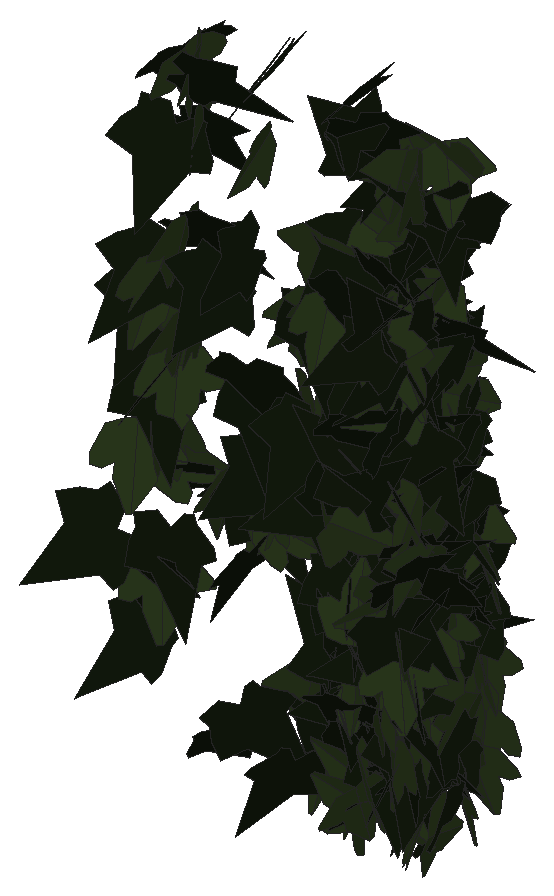
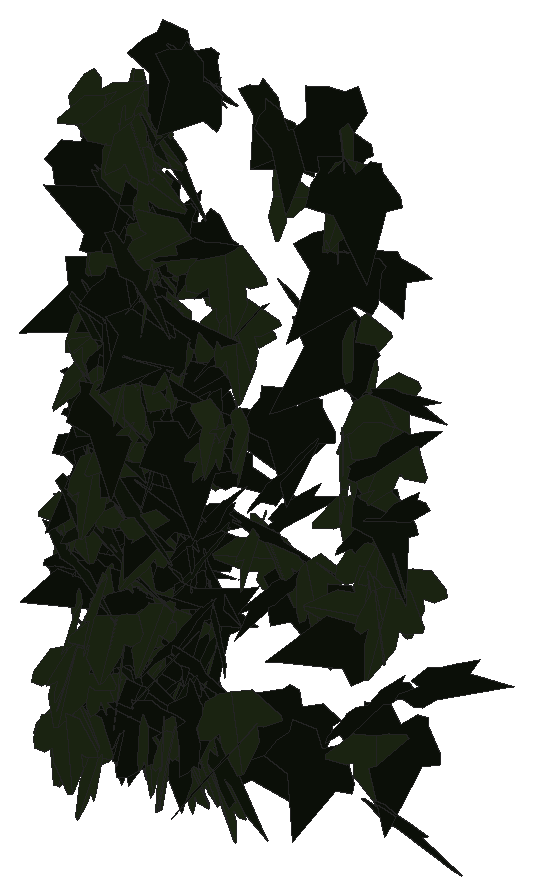
# SketchUp Ruby script. Lengths in inches.
U = 1.inch
M = Sketchup.active_model
def pt(a) = Geom::Point3d.new(a.map { |v| v * U })
def face(e, loops, mat)
  f = e.add_face(loops[0].map { |a| pt(a) })
  loops[1..].each { |l| e.add_face(l.map { |a| pt(a) }).erase! }
  f.material = f.back_material = mat if mat
  f
end
# faces: each face lists its corners as indices into pts; further lists are holes
def faces(e, pts, list, mat = nil) = list.each { |f| face(e, (f[0].is_a?(Array) ? f : [f]).map { |l| l.map { |i| pts[i] } }, mat) }
# xy, xz, yz: faces in a plane at the given z, y or x. An outline is a flat list of corners, or four numbers for a rectangle; further outlines are holes
def ring(l) = l.size == 4 ? [[l[0], l[1]], [l[2], l[1]], [l[2], l[3]], [l[0], l[3]]] : l.each_slice(2).to_a
def flat(e, list, mat, &to3) = list.each { |f| face(e, (f[0].is_a?(Array) ? f : [f]).map { |l| ring(l).map { |u, v| to3.(u, v) } }, mat) }
def xy(e, z, list, mat = nil) = flat(e, list, mat) { |x, y| [x, y, z] }
def xz(e, y, list, mat = nil) = flat(e, list, mat) { |x, z| [x, y, z] }
def yz(e, x, list, mat = nil) = flat(e, list, mat) { |y, z| [x, y, z] }
def lines(e, pts, list) = list.each { |a, b| e.add_line(pt(pts[a]), pt(pts[b])) }
# prism: a flat outline (further loops are holes) pulled along v
def prism(e, loops, v, mat = nil)
  f = face(e, loops, mat); d = Geom::Vector3d.new(v.map { |x| x * U })
  f.pushpull(f.normal.samedirection?(d) ? d.length : -d.length)
end
def box(e, o, s, mat = nil) = prism(e, [[o, [o[0] + s[0], o[1], o[2]], [o[0] + s[0], o[1] + s[1], o[2]], [o[0], o[1] + s[1], o[2]]]], [0, 0, s[2]], mat)
def at(x, y, z, deg = 0) = Geom::Transformation.translation(pt([x, y, z])) * Geom::Transformation.rotation(ORIGIN, Z_AXIS, deg.degrees)
def axes(o, x, y, z) = Geom::Transformation.new([*x, 0, *y, 0, *z, 0, *pt(o).to_a, 1])
def part(name) = M.definitions.add(name)
# library, detail: a bought-in or finely detailed component or shape, given as its bounding box
def library(name, o, s) = part(name).tap { |d| box(d.entities, o, s) }
def detail(e, o, s) = box(e.add_group.entities, o, s)
def put(e, d, t, mat = nil) = e.add_instance(d, t).tap { |i| i.material = mat if mat }
def group(e, t, mat = nil) = e.add_group.tap { |g| g.transformation = t; g.material = mat if mat }.entities
root = M.entities
M.materials.add("efeu1").color = [18, 25, 13]
M.materials.add("efeu2").color = [43, 57, 29]
c1 = part("ivyleaf_9")
p = [[1.54,2.16,1.25],[1.36,2.04,1.19],[-0.21,0.99,0.68],[-0.71,1.11,0.82],[-0.85,0.86,0.67],[-0.8,0.17,0.21],
  [-0.9,-0.01,0.1],[-0.67,-0.16,-0.02],[-0.08,-0.08,-0.05],[-0.03,-0.6,-0.4],[0.65,-0.88,-0.66],[0.83,-0.6,-0.49],
  [1.29,-0.42,-0.43],[1.8125,-0.07,-0.26],[1.21,0.44,0.15]]
faces(c1.entities,p,[[0,1,2,3,4,5,6,7,8,9,10,11,12,13,14]],"efeu1")
c2 = part("ivyleaf_10")
p = [[0,0.5,-0.03],[-0.0625,2.02,-0.43],[-0.19,2.01,-0.46],[-0.54,1.05,-0.29],[-0.52,0.625,-0.18],[-0.83,0.76,-0.28],
  [-1.16,0.64,-0.33],[-1.15,0.33,-0.24],[-0.77,-0.39,0.02],[-0.3,-0.51,0.16],[0.04,-0.48,0.23],[-0.02,2.01,-0.4375],
  [-0.06,2.01,-0.43],[0.04,-0.49,0.23],[0.67,-0.49,0.14],[1.38,0.36,-0.2],[1.375,0.51,-0.24],[0.81,0.65,-0.19],
  [0.62,0.59,-0.15],[0.6,1.09,-0.28],[0.5,1.23,-0.31]]
faces(c2.entities,p,[[0,1,2,3,4,5,6,7,8,9,10],[11,12,0,13,14,15,16,17,18,19,20]],"efeu2")
put(root,c1,axes([2.26,224.04,225.46],[-0.33992,-0.24824,0.26986],[-0.17412,-0.21457,-0.4167],[0.3227,-0.37727,0.05943]))
put(root,c1,axes([2.4,224.73,223.76],[-0.49927,0.02483,-0.01047],[0.00793,-0.05019,-0.49741],[-0.02575,-0.49685,0.04972]))
put(root,c1,axes([2.41,224.39,224.89],[0.35781,0.24755,-0.24635],[-0.21533,-0.1213,-0.43465],[-0.27496,0.41714,0.0198]))
put(root,c2,axes([2.41,224.64,226.9],[-0.10833,-0.43935,-0.21269],[0.08333,0.19802,-0.45149],[0.48096,-0.13327,0.03032]))
put(root,c2,axes([2.68,224.61,227.07],[0.27047,-0.37993,-0.18027],[-0.08089,0.16333,-0.4656],[0.41268,0.28102,0.02689]))
put(root,c2,axes([2.55,224.69,224.7],[0.37414,0.33148,0.01172],[0.00935,0.00712,-0.49986],[-0.33156,0.37426,-0.00086]))
put(root,c2,axes([2.63,224.04,226.96],[0.42358,0.26564,-0.00356],[-0.00319,-0.00162,-0.49999],[-0.26565,0.42359,0.00033]))
put(root,c1,axes([2.74,224.42,229.04],[-0.21253,-0.4395,0.10803],[-0.03639,-0.10236,-0.48806],[0.45112,-0.21531,0.01152]))
put(root,c1,axes([3.02,223.99,228.01],[-0.17079,0.46892,0.03075],[-0.00354,0.03144,-0.499],[-0.46991,-0.17067,-0.00742]))
put(root,c2,axes([2.91,224.34,227.25],[-0.49705,0.04613,0.02857],[-0.03096,-0.02493,-0.49842],[-0.04456,-0.49724,0.02763]))
put(root,c1,axes([2.7,224.7,225.29],[0.04335,-0.49242,-0.07509],[-0.00716,0.07475,-0.49433],[0.49807,0.04393,-0.00057]))
put(root,c2,axes([2.96,224.12,227.24],[-0.17393,0.43653,0.17084],[-0.13153,0.12946,-0.46469],[-0.44994,-0.20659,0.0698]))
put(root,c1,axes([3.02,224.12,229.75],[-0.4399,-0.23646,0.02393],[0.03632,-0.11663,-0.48485],[0.23487,-0.42484,0.11979]))
put(root,c2,axes([2.88,224.1,229.02],[-0.44475,-0.18072,-0.13976],[0.1366,0.03482,-0.47972],[0.18312,-0.46489,0.0184]))
put(root,c1,axes([2.87,224.22,227.9],[-0.00625,-0.48515,-0.12079],[-0.01142,0.1209,-0.48503],[0.49983,-0.0033,-0.0126]))
put(root,c2,axes([3.09,223.94,229.59],[0.20409,0.4084,-0.20385],[-0.1269,-0.16372,-0.45507],[-0.43845,0.23749,0.03683]))
put(root,c2,axes([2.77,224.45,226.53],[0.00807,-0.03471,0.49873],[0.43105,0.25315,0.01064],[-0.25324,0.42978,0.03401]))
put(root,c1,axes([2.82,224.54,226.32],[0.44308,0.01063,0.23144],[0.22107,0.13005,-0.4292],[-0.06932,0.48267,0.11055]))
put(root,c2,axes([3.11,224.3125,228.08],[0.31685,0.38417,-0.04498],[-0.03416,-0.03013,-0.49792],[-0.38528,0.3186,0.00715]))
put(root,c1,axes([3.35,224.15,233.01],[0.01762,0.49548,-0.06469],[-0.05228,-0.06255,-0.49331],[-0.49695,0.02415,0.04961]))
put(root,c1,axes([3.21,224.11,231.76],[-0.38608,-0.29312,-0.12255],[0.09909,0.07214,-0.48474],[0.30186,-0.39859,0.00239]))
put(root,c2,axes([3.26,224.27,228.88],[0.04513,-0.49718,-0.02777],[0.00392,0.02824,-0.49919],[0.49794,0.04484,0.00644]))
put(root,c2,axes([3.38,224.36,228.92],[0.20097,-0.39637,-0.22913],[-0.02558,0.24012,-0.43782],[0.45712,0.1877,0.07624]))
put(root,c2,axes([3.42,224.02,230.4],[0.06062,-0.49609,0.01495],[0.01955,-0.01266,-0.49946],[0.49593,0.06114,0.01786]))
put(root,c1,axes([3.26,224.29,231.83],[0.46235,0.1903,0.00424],[0.00518,-0.00145,-0.49997],[-0.19027,0.46237,-0.00332]))
put(root,c2,axes([3.47,224.09,232.91],[-0.16037,-0.41396,-0.23004],[0.10967,0.20381,-0.44321],[0.46071,-0.19261,0.02543]))
put(root,c2,axes([3.73,223.97,232.07],[-0.1549,0.42725,0.20849],[-0.26925,0.10187,-0.40881],[-0.3918,-0.23892,0.19851]))
put(root,c1,axes([3.47,224.12,230.39],[0.47347,0.14341,0.0725],[0.0648,0.03605,-0.49447],[-0.14705,0.47763,0.01555]))
put(root,c2,axes([3.81,223.8,233.15],[0.22729,-0.43822,-0.07937],[0.0098,0.09401,-0.49099],[0.44525,0.22164,0.05132]))
put(root,c2,axes([3.9,224.42,226.68],[0.05666,-0.49677,-0.00238],[-0.00053,0.00234,-0.49999],[0.49678,0.05666,-0.00027]))
put(root,c1,axes([4.08,224.09,229.77],[-0.22286,-0.3816,0.23391],[0.00769,-0.26453,-0.42422],[0.44752,-0.18549,0.12377]))
put(root,c1,axes([4.42,223.59,223.47],[0.16265,0.40557,0.04719],[0.02659,0.03925,-0.44983],[-0.43994,0.15232,-0.00974]))
put(root,c1,axes([4.06,223.4,233.14],[0.44335,0.04612,0.22652],[0.22564,0.02018,-0.44574],[-0.05026,0.49746,-0.00292]))
put(root,c1,axes([4.69,223.84,230.5625],[-0.44518,0.11169,-0.086],[0.08585,-0.02281,-0.44415],[-0.1231,-0.4198,0.00125]))
put(root,c1,axes([4.31,224.49,226.55],[0.16793,-0.41956,-0.21393],[-0.00025,0.22705,-0.44548],[0.47096,0.14972,0.07605]))
put(root,c1,axes([4.96,224.46,227.18],[-0.45656,0.1186,0.16579],[-0.18044,-0.04595,-0.46404],[-0.09484,-0.48355,0.08476]))
put(root,c1,axes([4.75,223.74,226.1],[-0.14471,0.36375,-0.20527],[0.07559,-0.18455,-0.40315],[-0.44052,-0.15116,-0.00175]))
put(root,c1,axes([4.78,223.85,233.08],[-0.06579,0.3891,0.19208],[-0.01428,0.18475,-0.40934],[-0.46495,-0.06073,-0.01461]))
put(root,c1,axes([4.66,223.83,228.81],[0.32779,0.22367,-0.22565],[-0.18782,-0.12974,-0.39211],[-0.27926,0.34981,-0.00115]))
put(root,c1,axes([4.43,224.33,228.15],[0.07692,-0.49391,0.01152],[-0.0076,-0.01284,-0.49978],[0.49399,0.07671,-0.00948]))
put(root,c1,axes([4.8,224.06,227.16],[-0.21161,-0.24551,0.31297],[-0.13765,-0.27775,-0.32196],[0.39622,-0.22761,0.0553]))
put(root,c2,axes([4.85,224.0625,226.75],[0.42955,-0.14661,-0.10158],[-0.09536,0.0428,-0.44074],[0.16463,0.40731,0.00975]))
put(root,c2,axes([4.85,223.95,232.14],[-0.07874,0.19352,-0.39801],[-0.08017,-0.38802,-0.18936],[-0.45616,0.03479,0.10198]))
put(root,c1,axes([4.96,223.8125,233.24],[0.0911,0.29753,0.31816],[-0.01364,0.31344,-0.31342],[-0.46068,0.04956,0.0722]))
put(root,c1,axes([4.85,223.51,223.96],[-0.04578,-0.12272,-0.43178],[0.14281,0.39355,-0.13503],[0.44522,-0.13886,-0.00109]))
put(root,c2,axes([5.05,224.18,226.94],[-0.15635,0.40635,0.05835],[-0.02651,0.05081,-0.44858],[-0.44222,-0.14671,0.00626]))
put(root,c2,axes([5.28,224.41,224.2],[-0.31464,-0.31848,0.05623],[-0.03611,-0.04269,-0.44887],[0.347,-0.29322,0.00428]))
put(root,c2,axes([5.15,224.375,228.47],[-0.26711,0.29156,-0.21578],[0.10472,-0.18818,-0.39521],[-0.37202,-0.26231,0.04369]))
put(root,c1,axes([5.41,224.51,223.39],[-0.34283,0.23911,-0.18396],[0.14872,-0.11116,-0.41327],[-0.28472,-0.34597,0.00564]))
put(root,c2,axes([4.92,223.98,226.49],[0.09282,0.01907,0.44304],[0.42676,0.1598,-0.09035],[-0.17312,0.40414,0.01482]))
put(root,c1,axes([5.14,224.7,223.66],[0.28128,-0.3725,-0.17923],[-0.05231,0.18297,-0.46237],[0.41005,0.27887,0.06396]))
put(root,c2,axes([5.54,224.48,228.54],[0.07507,0.17716,0.40681],[-0.28386,0.33091,-0.10729],[-0.36674,-0.21986,0.16631]))
put(root,c2,axes([5.47,224.08,229.875],[-0.02902,-0.49379,-0.07302],[0.00703,0.07273,-0.49463],[0.49911,-0.02974,0.00273]))
put(root,c2,axes([5.39,224.54,223.06],[0.40203,-0.22472,0.01308],[0.01328,-0.00397,-0.4522],[0.24271,0.37244,0.00307]))
put(root,c1,axes([5.57,223.64,223.32],[-0.04818,0.25155,-0.36616],[0.02111,-0.35241,-0.26444],[-0.46685,-0.04189,0.02583]))
put(root,c2,axes([5.56,224.16,229.99],[-0.23399,-0.43296,0.08831],[-0.01094,-0.09422,-0.49092],[0.44174,-0.23167,0.03462]))
put(root,c2,axes([5.6875,224.12,230.85],[-0.47361,-0.09232,0.13103],[-0.12689,-0.03378,-0.48245],[0.09793,-0.49024,0.00857]))
put(root,c2,axes([5.52,224.46,228.32],[-0.04509,0.41578,0.1257],[-0.00059,0.12137,-0.43443],[-0.46763,-0.04024,-0.01157]))
put(root,c1,axes([5.73,223.8,228.29],[-0.40757,-0.20368,-0.07589],[0.0698,0.03389,-0.44599],[0.223,-0.38287,0.0009]))
put(root,c1,axes([5.51,224.15,229.75],[0.10925,-0.48418,0.06029],[0.01544,-0.05832,-0.49635],[0.48767,0.11031,0.00221]))
put(root,c1,axes([5.875,224.62,228.23],[0.06639,0.42206,-0.08893],[-0.01441,-0.08446,-0.44357],[-0.46486,0.0629,0.00105]))
put(root,c2,axes([5.93,225.01,223.7],[-0.289,0.25274,0.2411],[-0.17101,0.16978,-0.38258],[-0.32856,-0.31068,-0.01294]))
put(root,c1,axes([6.19,223.71,227.4],[-0.40656,-0.02731,0.22492],[-0.23282,-0.01735,-0.39253],[0.03491,-0.4338,0.00154]))
put(root,c1,axes([6.24,224.47,229.82],[-0.11263,0.17983,0.3974],[-0.37704,0.18477,-0.18952],[-0.25665,-0.35035,0.10402]))
put(root,c1,axes([5.59,224.86,224],[0.12589,-0.03447,-0.43438],[0.45055,-0.03188,0.12381],[-0.04325,-0.43246,0.0255]))
put(root,c1,axes([6.07,223.7,224.7],[0.07921,-0.04203,0.44378],[-0.0227,0.43203,0.04801],[-0.46252,-0.0284,0.07365]))
put(root,c2,axes([6.21,223.94,223.01],[0.16723,-0.11354,-0.40594],[-0.26434,0.30745,-0.19398],[0.35053,0.28602,0.04738]))
put(root,c1,axes([5.87,224.42,226.79],[-0.0248,-0.46236,0.18871],[0.00568,-0.18919,-0.46279],[0.49935,-0.02081,0.01463]))
put(root,c1,axes([6.18,224.4,230.93],[-0.35942,-0.25412,0.12261],[-0.09565,-0.07823,-0.43539],[0.28703,-0.34428,0.00844]))
put(root,c1,axes([6.36,223.8,225.14],[-0.41075,-0.17686,-0.11991],[-0.11293,-0.04859,0.43622],[-0.19809,0.39444,-0.00003]))
put(root,c2,axes([6.18,224.72,223.61],[0.30005,-0.25895,-0.30482],[-0.07663,0.33679,-0.36153],[0.39255,0.26367,0.16242]))
put(root,c1,axes([6.47,224.1,224.43],[-0.40017,0.14775,0.18044],[-0.18105,0.0476,-0.41451],[-0.16671,-0.40636,0.01705]))
put(root,c2,axes([6.49,223.9,222.63],[0.02,0.05692,0.4481],[-0.43169,0.17153,-0.0057],[-0.18426,-0.39568,0.06199]))
put(root,c2,axes([6.18,223.59,230.3125],[0.24398,0.35202,-0.12424],[-0.06042,-0.106,-0.43489],[-0.3969,0.23253,-0.01017]))
put(root,c2,axes([6.17,223.61,227.59],[-0.15293,0.40834,-0.05133],[0.0261,-0.04385,-0.44939],[-0.44344,-0.1434,-0.00875]))
put(root,c2,axes([6.18,224.4,229.3125],[-0.06502,0.42921,-0.03862],[0.00094,-0.03738,-0.45073],[-0.46528,-0.06006,0.00449]))
put(root,c2,axes([6.6,223.83,223.3125],[-0.13851,0.04076,-0.43021],[-0.43036,0.11114,0.13987],[0.12775,0.41858,0.00475]))
put(root,c1,axes([6.3,223.83,233.33],[0.15562,0.3036,0.28725],[0.03675,0.28288,-0.34185],[-0.44175,0.13049,0.07275]))
put(root,c1,axes([6.62,223.5,225.62],[-0.14839,0.01385,-0.429],[-0.44574,-0.00692,0.14273],[-0.00237,0.43472,0.01593]))
put(root,c1,axes([6.15,224.6,225.07],[0.03517,-0.47864,0.14025],[0.00779,-0.14006,-0.47992],[0.4987,0.03594,-0.00239]))
put(root,c2,axes([6.3,223.64,224.44],[-0.30533,0.32962,-0.0265],[0.01796,-0.01931,-0.45162],[-0.3566,-0.2832,-0.00005]))
put(root,c2,axes([6.59,223.93,222.87],[-0.27429,-0.09919,-0.3525],[-0.31739,-0.17216,0.28142],[-0.21151,0.38697,0.03484]))
put(root,c1,axes([6.46,224.65,227.25],[-0.4374,-0.11108,-0.11794],[0.12159,0.01809,-0.43658],[0.12086,-0.42019,0.01239]))
put(root,c1,axes([6.14,224.68,224.75],[0.22249,-0.44572,-0.04279],[0.00938,0.05241,-0.49716],[0.44767,0.22042,0.03169]))
put(root,c2,axes([6.32,224.73,226.71],[0.1111,0.28458,0.325],[-0.00287,0.32205,-0.3041],[-0.45646,0.06725,0.08101]))
put(root,c1,axes([6.16,223.9375,226.02],[0.15414,-0.39325,0.12397],[0.05374,-0.10872,-0.43498],[0.44053,0.15086,0.00969]))
put(root,c1,axes([6.42,224.52,227.21],[0.25875,0.36226,0.02531],[0.01293,0.02125,-0.45169],[-0.39191,0.23988,0.0018]))
put(root,c1,axes([6.72,224.91,229.14],[-0.4227,-0.0718,0.18276],[-0.18024,-0.06179,-0.41281],[0.09772,-0.42456,0.02917]))
put(root,c1,axes([6.14,223.89,228.04],[0.40739,-0.19975,0.08725],[0.08098,-0.03766,-0.4439],[0.21952,0.38459,0.00185]))
put(root,c1,axes([6.37,224.6,229.8],[0.35024,0.26565,0.12079],[0.0132,0.16158,-0.41984],[-0.31285,0.30421,0.11752]))
put(root,c1,axes([6.29,223.86,226.22],[-0.00017,-0.26258,-0.36068],[0.06804,0.34314,-0.27022],[0.46485,-0.05032,0.03942]))
put(root,c1,axes([6.27,223.96,224.21],[0.05284,-0.29798,0.32564],[0.07429,-0.30573,-0.31377],[0.46087,0.08345,0.01324]))
put(root,c1,axes([6.58,223.56,225.79],[0.00073,-0.06487,0.44734],[0.046,0.42808,0.06707],[-0.46754,0.04202,0.0073]))
put(root,c1,axes([6.6875,223.74,227.98],[-0.19782,-0.39314,-0.0347],[0.0043,-0.03862,0.45059],[-0.4261,0.18213,0.02065]))
put(root,c1,axes([6.66,224.33,229.52],[-0.38911,-0.22375,0.10058],[-0.0887,-0.05107,-0.44108],[0.24786,-0.36953,0.00006]))
put(root,c1,axes([6.42,224.13,223.12],[-0.30709,0.03174,0.34077],[0.33923,-0.10346,0.2939],[0.10644,0.42132,0.0465]))
put(root,c1,axes([6.69,224.72,223.8],[-0.47785,-0.14588,-0.01937],[0.01858,0.00547,-0.49962],[0.14598,-0.47822,0.00019]))
put(root,c2,axes([6.27,224.43,231.13],[0.20396,0.14138,0.38009],[0.28216,0.25695,-0.24378],[-0.31543,0.32126,0.02771]))
put(root,c1,axes([6.77,225.02,227.48],[-0.36396,0.26857,-0.06175],[0.04344,-0.04477,-0.44805],[-0.29386,-0.33925,0.01024]))
put(root,c1,axes([6.89,223.33,233.09],[-0.11577,0.24399,0.35756],[-0.29493,0.23008,-0.25836],[-0.34688,-0.27705,0.10033]))
put(root,c1,axes([6.64,223.55,225.21],[0.3109,0.01209,-0.33893],[-0.35221,0.01182,-0.29913],[0.00093,0.43467,0.01756]))
put(root,c1,axes([6.76,223.33,224.74],[0.17707,0.32611,-0.24609],[-0.28496,-0.10617,-0.34231],[-0.32887,0.26759,0.1641]))
put(root,c1,axes([6.57,223.73,224.0625],[0.38115,0.19828,-0.16561],[-0.1446,-0.08671,-0.42088],[-0.23351,0.37735,-0.0097]))
put(root,c1,axes([6.48,223.72,226.48],[-0.13285,-0.37565,-0.18886],[0.06842,0.17032,-0.41104],[0.4454,-0.13821,0.0068]))
put(root,c1,axes([6.84,224.76,230.95],[-0.28726,0.34399,0.01285],[-0.00684,0.01072,-0.45221],[-0.37168,-0.26605,-0.00161]))
put(root,c1,axes([6.23,223.58,230.48],[0.31426,0.09406,-0.32174],[0.2837,0.17393,0.31195],[0.20364,-0.38746,0.06192]))
put(root,c1,axes([6.89,223.96,232.375],[-0.29915,0.33145,0.05345],[-0.03436,0.0404,-0.44923],[-0.36061,-0.27881,-0.00154]))
put(root,c2,axes([6.61,224.54,223.51],[0.11246,-0.48716,0.00483],[0.0845,0.01462,-0.49259],[0.4798,0.11161,0.08562]))
put(root,c2,axes([6.75,224.41,230.36],[-0.26481,0.30327,0.2004],[-0.15765,0.12909,-0.40447],[-0.35459,-0.28388,0.03017]))
put(root,c1,axes([6.83,224.55,227.7],[-0.01612,0.3637,-0.2477],[-0.06436,-0.23778,-0.37373],[-0.46509,0.0203,0.06031]))
put(root,c1,axes([6.74,223.53,228.89],[0.22676,0.35625,-0.1404],[-0.10681,-0.09789,-0.42863],[-0.39735,0.22962,0.0351]))
put(root,c1,axes([6.72,224.36,227.53],[0.24426,-0.06509,-0.38047],[-0.35429,0.16619,-0.24166],[0.1885,0.3967,0.03881]))
put(root,c2,axes([6.64,224.36,225.14],[0.01279,0.41207,0.14443],[-0.02717,0.13934,-0.42776],[-0.46884,0.00317,0.02873]))
put(root,c1,axes([6.83,223.66,223.2],[0.03297,0.43352,-0.01958],[-0.03097,-0.01682,-0.45108],[-0.46762,0.03168,0.02849]))
put(root,c1,axes([7.04,224.58,226.59],[-0.1336,0.16359,0.39896],[-0.29401,0.27145,-0.21168],[-0.3412,-0.29796,0.02619]))
put(root,c1,axes([6.47,223.43,227.48],[-0.08647,-0.04399,0.44231],[0.46177,-0.00888,0.08275],[0.00069,0.43268,0.04667]))
put(root,c2,axes([6.8125,224.9,228.82],[-0.35761,-0.28042,0.03202],[-0.00986,-0.0368,-0.45068],[0.30451,-0.33051,0.02301]))
put(root,c2,axes([6.58,224.1,229.47],[-0.00398,-0.07163,0.44621],[0.13413,0.41103,0.07247],[-0.45023,0.12308,0.01765]))
put(root,c1,axes([6.46,223.87,232.875],[0.31352,-0.37895,-0.09],[0.04189,0.14767,-0.47585],[0.38723,0.29084,0.12435]))
put(root,c2,axes([7.1,224.14,232.35],[0.01138,0.04115,0.45024],[-0.46822,0.03496,0.00751],[-0.03684,-0.43164,0.04354]))
put(root,c1,axes([6.73,224.61,230.08],[0.33616,0.29722,-0.0658],[-0.04489,-0.04807,-0.44755],[-0.3251,0.31397,-0.00624]))
put(root,c2,axes([6.78,225,228.05],[0.2301,0.31324,-0.22236],[-0.12666,-0.1788,-0.39397],[-0.38951,0.24319,-0.00325]))
put(root,c2,axes([6.73,223.46,225.85],[0.24033,0.3544,-0.12353],[0.07229,0.09822,0.43519],[0.39715,-0.23233,-0.00446]))
put(root,c2,axes([7.125,224.24,231.78],[-0.07705,0.01298,0.44607],[-0.45916,-0.0611,-0.07163],[0.06284,-0.43049,0.02361]))
put(root,c2,axes([6.63,223.58,225.2],[0.40657,-0.15564,0.1587],[0.14903,-0.06557,-0.42358],[0.18222,0.40088,-0.00766]))
put(root,c1,axes([6.7,224.93,229.03],[-0.22778,-0.38037,0.00794],[0.07837,-0.04879,-0.44317],[0.40334,-0.20533,0.09059]))
put(root,c2,axes([6.625,223.76,224.71],[0.17303,0.33825,0.23055],[0.10302,0.20011,-0.38925],[-0.42445,0.18646,-0.00049]))
put(root,c2,axes([6.62,223.375,227.35],[-0.16831,-0.18703,-0.37492],[0.28126,0.25026,-0.25212],[0.33656,-0.30268,0.0232]))
put(root,c1,axes([6.8125,224.54,230.16],[0.21069,0.38763,-0.03144],[-0.01662,-0.0261,-0.4513],[-0.41958,0.19568,0.00208]))
put(root,c2,axes([6.81,223.43,223.37],[-0.14966,-0.38392,-0.15645],[0.05208,0.14252,-0.42448],[0.44227,-0.1467,-0.00296]))
put(root,c2,axes([6.72,223.91,224.84],[0.03178,-0.05007,0.44835],[0.03841,0.43092,0.04952],[-0.46715,0.03202,0.03457]))
put(root,c1,axes([6.95,225,228.57],[-0.00859,0.43415,0.02705],[0.00268,0.02605,-0.45158],[-0.46971,-0.00779,-0.00307]))
put(root,c1,axes([6.76,224.48,228.82],[-0.23806,0.10804,-0.37348],[0.34656,-0.16125,-0.25529],[-0.20961,-0.3893,0.00209]))
put(root,c2,axes([6.76,225.16,225.28],[0.21092,0.38215,0.07389],[0.00526,0.0771,-0.44521],[-0.41976,0.19298,0.03155]))
put(root,c2,axes([6.82,223.56,223.82],[-0.21922,0.38423,0.02065],[-0.00784,0.01862,-0.45192],[-0.41545,-0.2031,-0.00236]))
put(root,c1,axes([7.13,223.6,230.17],[-0.45516,0.01175,0.11138],[-0.11578,-0.00291,-0.43844],[-0.01152,-0.43483,0.00594]))
put(root,c1,axes([7.2,224.53,228.32],[-0.18933,0.31165,0.25764],[-0.22075,0.16183,-0.36215],[-0.36897,-0.25674,0.08447]))
put(root,c2,axes([6.91,225.28,225.82],[-0.21976,0.37411,0.09221],[-0.05315,0.07415,-0.44283],[-0.41182,-0.20921,0.00795]))
put(root,c1,axes([7.15,224.42,227.87],[-0.44514,-0.07379,0.12262],[-0.12434,-0.02592,-0.43544],[0.08429,-0.42791,0.00523]))
put(root,c1,axes([6.84,223.42,233.39],[0.36313,0.27234,-0.04655],[-0.03785,-0.02784,-0.45],[-0.29566,0.33805,0.00044]))
put(root,c2,axes([7.01,224.41,232.52],[0.03842,0.41562,-0.12831],[-0.161,-0.10451,-0.41087],[-0.43968,0.07458,0.13924]))
put(root,c1,axes([7.16,223.51,228.61],[-0.01688,0.17245,0.41501],[-0.11989,0.38449,-0.17732],[-0.45393,-0.10796,0.0314]))
put(root,c1,axes([6.81,224.0625,223.67],[0.01305,-0.4318,-0.05329],[-0.00315,0.05118,-0.44925],[0.46961,0.01234,-0.00153]))
put(root,c1,axes([6.83,223.73,231.16],[0.45134,-0.02071,-0.12371],[-0.12832,0.0058,-0.43516],[0.02323,0.43447,-0.00008]))
put(root,c2,axes([7.19,223.89,229.23],[0.22658,0.11086,-0.37917],[-0.37099,-0.12514,-0.24515],[-0.17815,0.40159,0.02828]))
put(root,c1,axes([6.63,224.5625,223.375],[0.23286,0.02806,0.39183],[0.40067,0.06632,-0.22594],[-0.07717,0.429,0.0093]))
put(root,c1,axes([6.77,223.83,225.11],[-0.15721,-0.00354,0.4263],[0.44247,0.01323,0.15143],[-0.01475,0.43478,-0.00114]))
put(root,c1,axes([6.8,223.87,224.91],[0.0759,0.03921,0.44459],[0.35648,0.27203,-0.08238],[-0.29644,0.33717,0.01477]))
put(root,c1,axes([7.01,223.95,223.64],[0.23073,0.378,-0.02754],[-0.01493,-0.0226,-0.45156],[-0.40897,0.21408,0.00095]))
put(root,c1,axes([6.83,223.97,224.34],[-0.24615,-0.13727,-0.35792],[0.32105,0.17344,-0.27668],[0.23886,-0.37457,0.00305]))
put(root,c1,axes([7.1,223.84,230.08],[0.2374,0.07091,0.38336],[-0.381,-0.10696,0.24018],[0.13855,-0.41564,0.00359]))
put(root,c2,axes([7.26,223.32,224.78],[-0.14659,0.17459,0.38958],[-0.35382,0.19491,-0.21793],[-0.2721,-0.3475,0.0735]))
put(root,c1,axes([7.375,224.47,225.96],[-0.30485,0.24053,0.23646],[-0.21116,0.11994,-0.38439],[-0.28843,-0.34203,0.03149]))
put(root,c1,axes([7.25,223.64,229.87],[-0.43494,0.15469,-0.05804],[0.05466,-0.02387,-0.44864],[-0.16898,-0.40587,0.00426]))
put(root,c2,axes([7.09,225.14,227.58],[-0.1048,-0.38282,-0.18965],[0.04324,0.17797,-0.4107],[0.45592,-0.10487,-0.00464]))
put(root,c2,axes([7.18,224.29,231.73],[-0.23069,-0.28218,-0.26304],[-0.1658,-0.20101,0.36807],[-0.37417,0.26305,-0.00092]))
put(root,c1,axes([7.39,223.75,225.47],[-0.3755,-0.02494,0.27063],[-0.26801,-0.10466,-0.35526],[0.08876,-0.42149,0.0722]))
put(root,c1,axes([6.97,224.55,223.375],[-0.03546,0.03224,-0.44986],[0.34354,-0.29313,-0.04784],[-0.31849,-0.31978,-0.00151]))
put(root,c2,axes([7.14,223.96,232.68],[-0.18881,-0.38951,0.08668],[0.00549,-0.0932,-0.44186],[0.43015,-0.16978,0.04369]))
put(root,c2,axes([7.02,224.78,228.87],[-0.32439,0.28574,-0.13704],[0.10605,-0.08795,-0.43113],[-0.32286,-0.31598,-0.00392]))
put(root,c2,axes([7.25,225.62,223.71],[-0.45823,0.0432,0.08908],[-0.09982,-0.08005,-0.43416],[-0.02775,-0.42538,0.09075]))
put(root,c1,axes([7.31,224.61,229.0625],[-0.15673,-0.35869,0.20671],[0.07937,0.18468,0.40241],[-0.43571,0.16267,-0.00105]))
put(root,c1,axes([7.39,223.93,226.71],[-0.25234,0.41409,-0.12189],[0.02,-0.12982,-0.48244],[-0.43119,-0.24835,0.04896]))
put(root,c2,axes([7.44,223.74,226.33],[0.0319,0.1864,-0.46286],[-0.41253,-0.25107,-0.12955],[-0.28072,0.39015,0.13777]))
put(root,c2,axes([6.92,223.92,223.21],[-0.25698,0.05071,-0.37503],[0.36544,-0.12842,-0.25098],[-0.14536,-0.41251,0.03203]))
put(root,c1,axes([7.44,224.75,228.42],[-0.22796,0.37053,-0.08934],[-0.05299,-0.12395,-0.43063],[-0.40735,-0.19123,0.10601]))
put(root,c2,axes([7.5,225.08,223.8],[-0.04687,0.08347,0.44169],[-0.43562,0.14703,-0.07291],[-0.16956,-0.4008,0.06523]))
put(root,c2,axes([7.15,223.67,226.55],[-0.39217,-0.17762,-0.16712],[0.14975,0.08209,-0.42022],[0.21094,-0.38851,-0.01238]))
put(root,c2,axes([7.1875,225.0625,223],[-0.34468,0.29518,-0.01601],[0.01365,-0.009,-0.45211],[-0.31894,-0.31939,-0.00205]))
put(root,c1,axes([7.29,224.16,230.82],[-0.13074,-0.24073,0.35516],[0.16247,0.30658,0.28022],[-0.42098,0.19308,-0.00215]))
put(root,c1,axes([7.06,224.83,228.4],[-0.17267,-0.30759,-0.27329],[0.1819,0.20629,-0.35771],[0.39725,-0.22816,0.04501]))
put(root,c2,axes([7.12,223.69,230.1875],[0.45091,-0.11668,-0.03746],[0.04244,0.0069,0.45049],[-0.12487,-0.419,0.01785]))
put(root,c2,axes([7.35,224.35,230.71],[0.28045,0.24435,-0.25914],[-0.24799,-0.11426,-0.3654],[-0.28383,0.34127,0.06321]))
put(root,c1,axes([7.45,223.63,223.96],[0.12898,-0.00182,-0.43501],[-0.45159,0.01115,-0.12421],[0.01212,0.43485,0.00136]))
put(root,c1,axes([7.29,224.16,224.66],[0.1055,0.27266,0.33754],[0.04365,0.32556,-0.29709],[-0.45572,0.0943,0.04968]))
put(root,c1,axes([7.41,223.71,230.78],[0.00853,0.41604,0.13186],[-0.05339,0.12684,-0.42967],[-0.46668,-0.00691,0.05156]))
put(root,c2,axes([7.2,224.52,225.84],[-0.10014,0.47705,-0.11132],[0.00814,-0.11198,-0.48723],[-0.4898,-0.09939,0.01466]))
put(root,c1,axes([7.66,224.17,225.05],[-0.26913,0.15432,0.39211],[-0.40999,0.01159,-0.28596],[-0.09735,-0.47545,0.1203]))
put(root,c2,axes([7.29,224.69,224.23],[0.00491,-0.48513,0.12095],[0.01922,-0.12068,-0.48484],[0.49961,0.00941,0.01746]))
put(root,c1,axes([7.43,224.22,226.34],[-0.01435,-0.11873,-0.435],[-0.05655,-0.41499,0.12423],[-0.46616,0.054,-0.00168]))
put(root,c2,axes([7.26,225.41,224.65],[-0.32577,-0.29982,-0.09502],[0.09251,0.04311,-0.44127],[0.32561,-0.31221,0.03031]))
put(root,c2,axes([7.36,224.3125,230.71],[-0.19622,-0.38973,0.06839],[-0.03194,-0.05877,-0.4472],[0.42567,-0.18406,-0.00203]))
put(root,c2,axes([7.28,224.21,224.26],[0.17872,-0.41519,-0.21372],[0.03985,0.24157,-0.43596],[0.46527,0.13879,0.11943]))
put(root,c1,axes([7.57,224.82,227.87],[-0.07017,-0.11047,-0.43232],[-0.21072,-0.3671,0.13317],[-0.41399,0.20558,0.00549]))
put(root,c2,axes([7.41,223.91,226.27],[-0.10549,0.31835,0.29108],[-0.20437,0.22427,-0.33397],[-0.40965,-0.19386,0.09166]))
put(root,c2,axes([7.26,225.44,224.82],[-0.1299,0.4172,0.02753],[-0.00613,0.02591,-0.45156],[-0.45144,-0.1204,-0.00179]))
put(root,c1,axes([7.17,224.31,228.45],[0.28952,0.29387,0.18311],[0.13856,0.12117,-0.4135],[-0.34306,0.29695,-0.01248]))
put(root,c1,axes([7.39,223.16,223.625],[0.06264,0.17876,0.408],[0.02122,0.39434,-0.18989],[-0.46512,0.04206,0.04629]))
put(root,c2,axes([7.27,225.34,225.39],[-0.21576,0.38243,-0.05756],[0.00151,-0.06158,-0.44784],[-0.41732,-0.19794,0.02813]))
put(root,c1,axes([7.62,224.25,226.71],[-0.08269,0.29955,0.31823],[-0.25357,0.23059,-0.29586],[-0.38675,-0.21523,0.12594]))
put(root,c2,axes([7.34,223.5625,224.8],[0.00926,0.26303,0.36022],[-0.10539,0.33876,-0.26503],[-0.45773,-0.07268,0.06831]))
put(root,c1,axes([7.57,224.75,229.78],[-0.36879,0.26886,-0.0191],[0.01022,-0.01766,-0.45192],[-0.29086,-0.34151,0.00834]))
put(root,c1,axes([7.57,224.92,227.05],[-0.32017,0.3122,-0.06472],[0.01477,-0.07247,-0.44585],[-0.34349,-0.29412,0.04116]))
put(root,c2,axes([7.3,225.15,226.96],[0.42303,0.18788,-0.02318],[-0.04041,0.02669,-0.44987],[-0.2003,0.39142,0.04181]))
put(root,c1,axes([7.52,224.72,228.8125],[-0.41076,-0.18748,0.10094],[-0.08916,-0.05198,-0.44088],[0.20985,-0.38907,0.01026]))
put(root,c1,axes([7.48,224.64,224.84],[-0.36861,0.17763,-0.21106],[0.16976,-0.13498,-0.39779],[-0.23669,-0.37344,0.04339]))
put(root,c2,axes([7.47,223.48,224.25],[-0.3818,0.24223,0.07764],[-0.13772,-0.05925,-0.42811],[-0.23658,-0.35643,0.12392]))
put(root,c2,axes([7.41,224.6875,229.58],[-0.20793,-0.38906,-0.0293],[0.02954,0.01787,-0.45112],[0.42024,-0.19375,0.01721]))
put(root,c2,axes([7.75,224.07,225.35],[-0.14178,0.03876,0.47791],[-0.44765,-0.18926,-0.11745],[0.17179,-0.46117,0.08837]))
put(root,c1,axes([7.36,224.07,227.85],[0.2244,0.35813,0.13874],[0.07402,0.11446,-0.4306],[-0.40605,0.21879,-0.00183]))
put(root,c1,axes([7.11,224.01,229.88],[0.19887,-0.35467,0.1787],[0.11246,-0.13913,-0.41473],[0.41051,0.20994,0.02704]))
put(root,c1,axes([7.56,224.375,231.71],[-0.42015,0.07989,-0.18459],[0.14175,-0.18524,-0.3859],[-0.15523,-0.38539,0.14722]))
put(root,c1,axes([7.36,224.62,225.87],[-0.16487,-0.40728,0.00696],[-0.00259,-0.00625,-0.45235],[0.43991,-0.15268,-0.00005]))
put(root,c1,axes([7.35,224.14,224.04],[-0.14168,-0.47949,0.00383],[-0.00125,-0.00362,-0.49999],[0.4795,-0.14169,-0.00018]))
put(root,c1,axes([7.18,223.81,226.88],[0.3124,0.04509,0.33461],[0.27549,0.23527,-0.2728],[-0.21731,0.3631,0.13521]))
put(root,c1,axes([7.11,225.08,226.92],[0.17705,-0.34058,0.22392],[0.19524,-0.14557,-0.38262],[0.3889,0.22813,0.09014]))
put(root,c1,axes([7.23,224.3,226.45],[0.46077,0.08078,0.02706],[0.02769,0.00446,-0.45159],[-0.08738,0.42741,-0.0004]))
put(root,c1,axes([7.72,225.02,226.24],[-0.30751,0.31852,0.08511],[-0.07113,0.05082,-0.44405],[-0.34798,-0.29187,0.01555]))
put(root,c1,axes([7.32,223.66,227.85],[0.40861,-0.1139,-0.18924],[-0.17889,0.07965,-0.41003],[0.14748,0.4122,0.02694]))
put(root,c1,axes([7.49,224.6,223.91],[-0.24023,-0.33975,0.16219],[-0.08778,-0.13318,-0.4223],[0.39408,-0.23677,0.00481]))
put(root,c2,axes([7.74,224.41,232.59],[-0.30132,0.02687,-0.34596],[-0.35911,-0.05963,0.28502],[-0.03097,0.43006,0.06113]))
put(root,c2,axes([7.54,223.75,223.09],[0.23533,-0.34415,-0.15876],[-0.08838,0.12887,-0.42363],[0.39689,0.23275,-0.00019]))
put(root,c1,axes([7.08,224.63,223.5625],[0.15079,-0.25882,0.40034],[0.29778,-0.27676,-0.29109],[0.37228,0.32621,0.07068]))
put(root,c2,axes([7.39,224.24,225.83],[-0.46348,-0.08987,-0.16465],[0.17022,-0.01715,-0.46982],[0.07879,-0.49156,0.04649]))
put(root,c1,axes([7.24,224.36,231.06],[0.00573,-0.01846,0.45196],[0.42579,0.18381,0.00311],[-0.19846,0.39383,0.01973]))
put(root,c2,axes([7.45,224.7,229],[-0.00521,0.19505,0.40434],[-0.05971,0.38539,-0.20179],[-0.46596,-0.05156,0.02134]))
put(root,c1,axes([7.23,224.0625,228.47],[-0.11042,-0.20243,-0.38606],[0.26591,0.28197,-0.23044],[0.37123,-0.26219,0.05023]))
put(root,c2,axes([7.53,224.39,227.34],[0.00944,-0.49986,0.00685],[-0.01671,-0.00716,-0.49967],[0.49963,0.00921,-0.01684]))
put(root,c2,axes([7.48,225.06,223.47],[-0.45799,-0.07062,-0.06905],[0.0699,0.01551,-0.44707],[0.07793,-0.42895,-0.0048]))
put(root,c1,axes([7.59,224.9,225.74],[-0.40211,-0.22471,-0.01052],[0.00971,0.00468,-0.45228],[0.24274,-0.37244,0.00067]))
put(root,c2,axes([7.22,223.73,229.96],[0.36342,0.03003,0.28499],[0.295,0.02203,-0.35134],[-0.04018,0.4334,-0.00189]))
put(root,c2,axes([7.49,223.68,227.84],[0.38197,-0.25223,-0.02359],[-0.02018,0.01288,-0.45178],[0.27276,0.35417,-0.00038]))
put(root,c1,axes([7.39,224.93,226.01],[-0.25908,-0.30516,-0.20421],[0.17613,0.11961,-0.40053],[0.35009,-0.286,0.05038]))
put(root,c1,axes([7.58,224.4,227.22],[-0.01834,0.12759,-0.4831],[-0.29219,0.38941,0.11394],[0.40532,0.2865,0.06028]))
put(root,c2,axes([7.46,224.17,224.26],[0.04964,0.42848,-0.06166],[-0.0179,-0.05783,-0.44805],[-0.46683,0.04778,0.01063]))
put(root,c2,axes([7.36,224.46,225.9375],[0.37976,-0.17583,0.19363],[0.17907,-0.0847,-0.40886],[0.21077,0.38876,-0.0015]))
put(root,c1,axes([7.7,224.66,228.8],[-0.4045,0.19438,-0.10989],[0.10468,-0.04259,-0.4388],[-0.21479,-0.38682,-0.00691]))
put(root,c1,axes([7.25,223.89,225.35],[0.00909,-0.03622,-0.45074],[0.46268,-0.07402,0.01509],[-0.08095,-0.42712,0.03561]))
put(root,c1,axes([7.6,223.7,226.78],[0.31516,0.30795,-0.23632],[-0.18114,-0.15254,-0.44036],[-0.34331,0.36318,0.01541]))
put(root,c1,axes([7.65,224.55,229.96],[-0.39743,0.14186,-0.19088],[0.18157,-0.07405,-0.41008],[-0.17262,-0.4045,0.00813]))
put(root,c2,axes([7.5,223.52,225.84],[-0.18673,0.39806,-0.0308],[0.01274,-0.02716,-0.45135],[-0.43091,-0.1733,0]))
put(root,c1,axes([7.49,224.15,226.67],[-0.16559,-0.47044,0.03559],[-0.01128,-0.03376,-0.49873],[0.47165,-0.16597,0.00056]))
put(root,c1,axes([7.79,223.375,229.37],[-0.16894,0.37557,0.16011],[-0.06856,0.14032,-0.4231],[-0.43298,-0.16876,0.00452]))
put(root,c1,axes([7.5,224.1875,224.03],[0.26748,-0.34691,-0.09031],[0.05547,-0.07002,0.44329],[-0.38222,-0.25293,0.00114]))
put(root,c1,axes([7.83,223.89,223.1],[-0.10615,0.31529,0.29445],[-0.11838,0.26183,-0.34281],[-0.44208,-0.14582,0.0211]))
put(root,c2,axes([7.6,224.35,227.59],[0.09533,-0.46528,0.15629],[0.02987,-0.15342,-0.47494],[0.48992,0.09989,-0.00145]))
put(root,c2,axes([7.6,223.64,232.7],[0.15319,-0.41123,-0.23964],[0.00823,0.25399,-0.4306],[0.47588,0.12799,0.08459]))
put(root,c2,axes([7.46,223.46,225.5],[0.39297,0.23027,0.06415],[0.05484,0.03511,-0.44782],[-0.25156,0.36738,0.00259]))
put(root,c1,axes([7.38,224.49,225.6],[0.27601,0.16794,0.32175],[0.25087,0.2068,-0.31631],[-0.28565,0.34388,0.03309]))
put(root,c1,axes([7.3,224.6,230],[0.44366,0.00862,0.14854],[0.15141,0.06258,-0.42329],[-0.0309,0.43039,0.05857]))
put(root,c1,axes([7.44,223.29,226.27],[-0.01531,-0.13206,-0.4308],[0.04217,0.41239,-0.13812],[0.46765,-0.04151,-0.00165]))
put(root,c1,axes([7.6,223.29,226.93],[0.1953,0.37428,0.13335],[0.07134,0.11044,-0.43215],[-0.42128,0.19221,-0.01135]))
put(root,c1,axes([7.42,224.4,231.84],[0.05743,-0.42649,0.06981],[0.06942,-0.05905,-0.4432],[0.46108,0.06201,0.05803]))
put(root,c1,axes([7.96,224.02,224.14],[-0.30153,0.28761,0.17574],[-0.13374,0.11525,-0.41679],[-0.33452,-0.30533,0.00822]))
put(root,c2,axes([7.71,223.71,227.1],[-0.05138,-0.38628,0.20207],[-0.02048,-0.19342,-0.40474],[0.46653,-0.05103,0.00449]))
put(root,c1,axes([7.59,223.79,225.99],[0.15751,0.14606,0.39823],[0.16347,0.3585,-0.20217],[-0.41132,0.19841,0.07214]))
put(root,c2,axes([7.66,224.63,224.42],[0.09644,-0.42208,0.25009],[0.05139,-0.24478,-0.43294],[0.48791,0.10922,-0.00383]))
put(root,c2,axes([7.7,223.88,222.93],[-0.00817,-0.16252,-0.41956],[0.01416,0.40322,-0.16919],[0.46952,-0.01499,-0.0022]))
put(root,c1,axes([7.8125,224.48,232.11],[-0.01276,0.17754,-0.41282],[-0.00915,-0.39711,-0.18446],[-0.46954,0.00291,0.01481]))
put(root,c2,axes([7.59,224.32,232.74],[0.24705,0.36994,0.00713],[0.00356,0.00602,-0.45234],[-0.39958,0.22877,0.00037]))
put(root,c2,axes([7.62,224.97,226.7],[-0.33437,0.29594,-0.07913],[0.06517,-0.04696,-0.44536],[-0.32351,-0.31534,-0.00794]))
